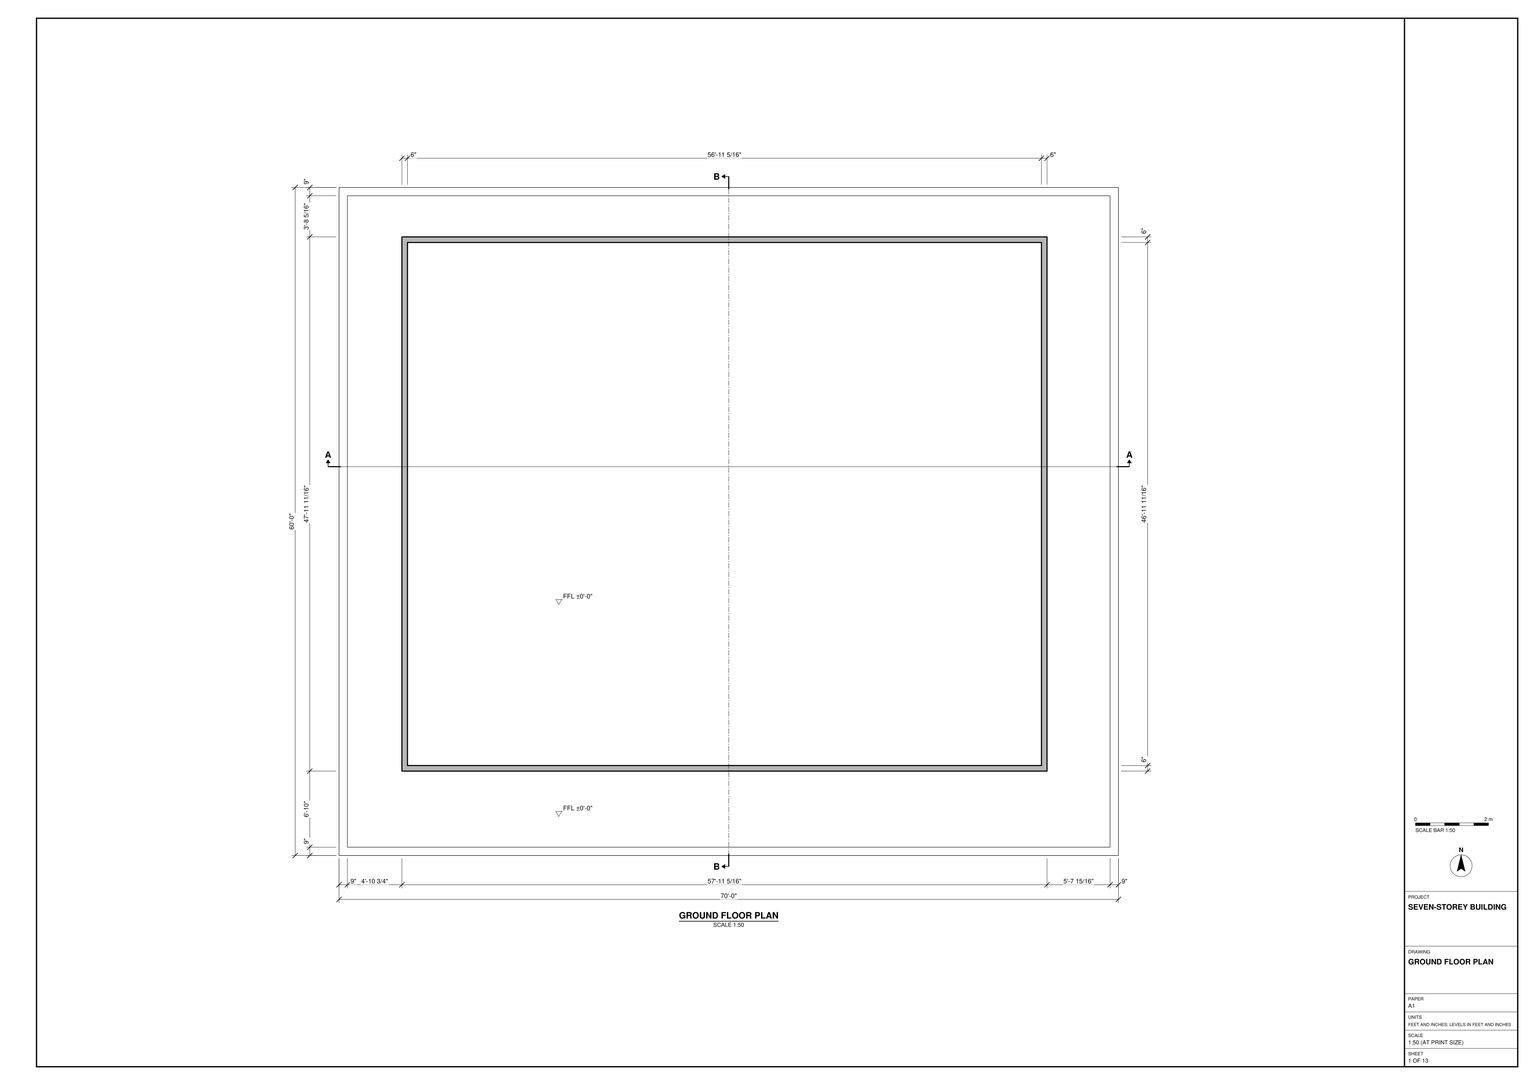
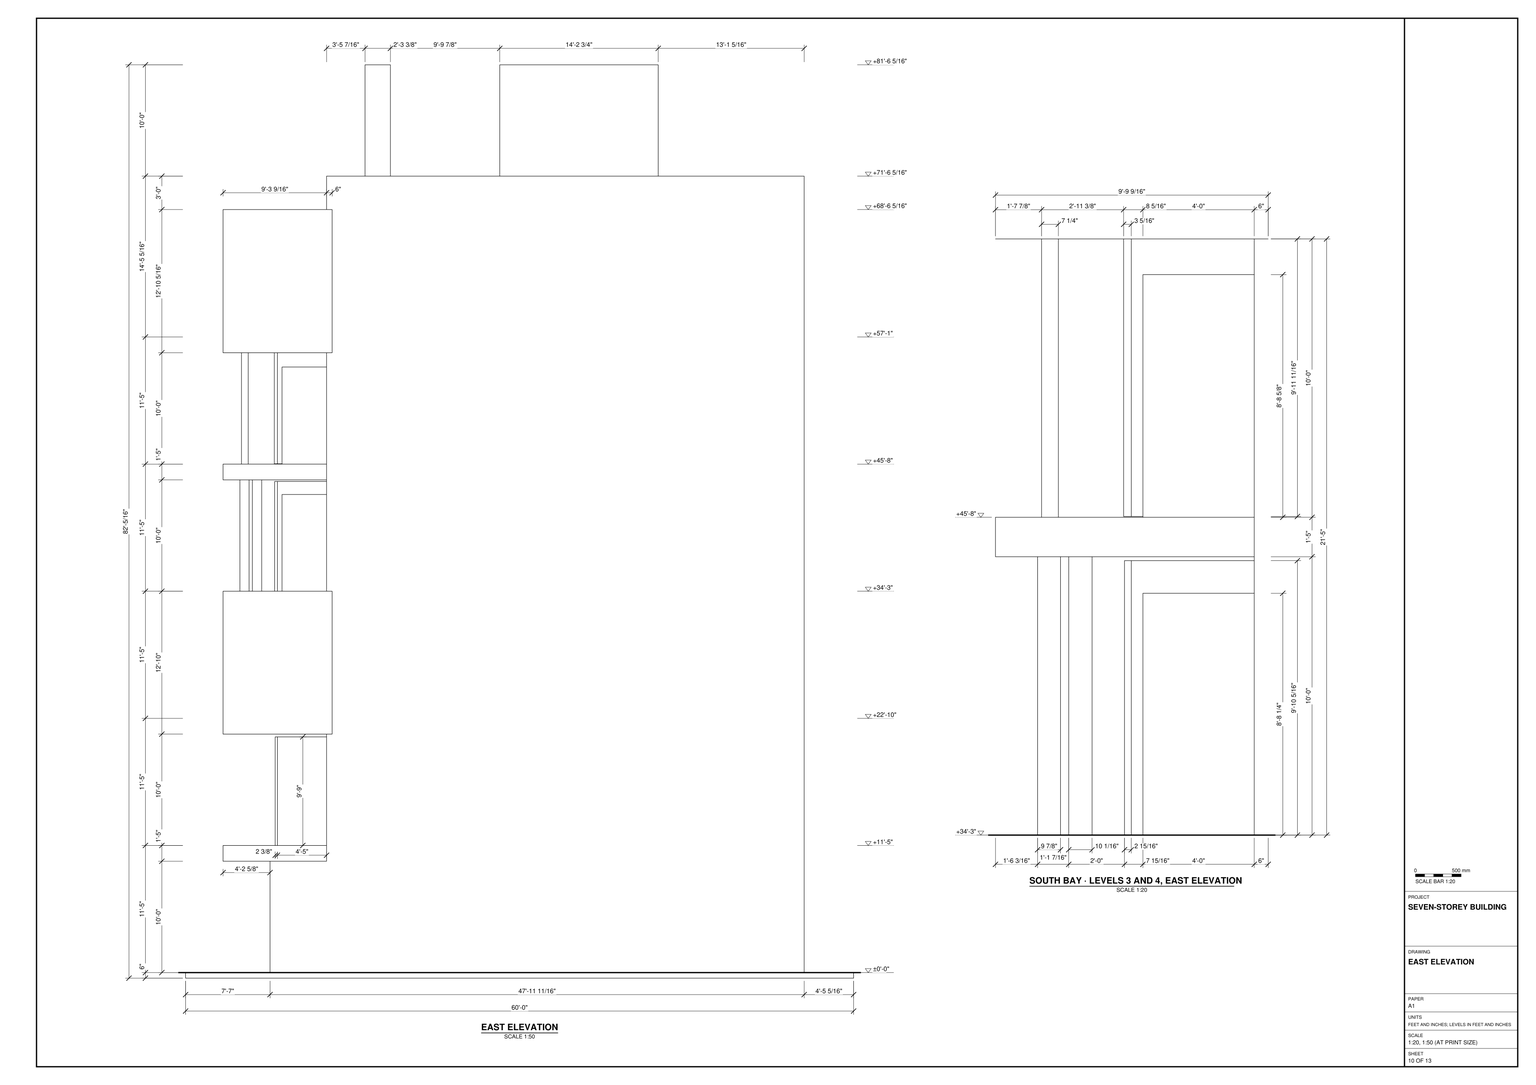
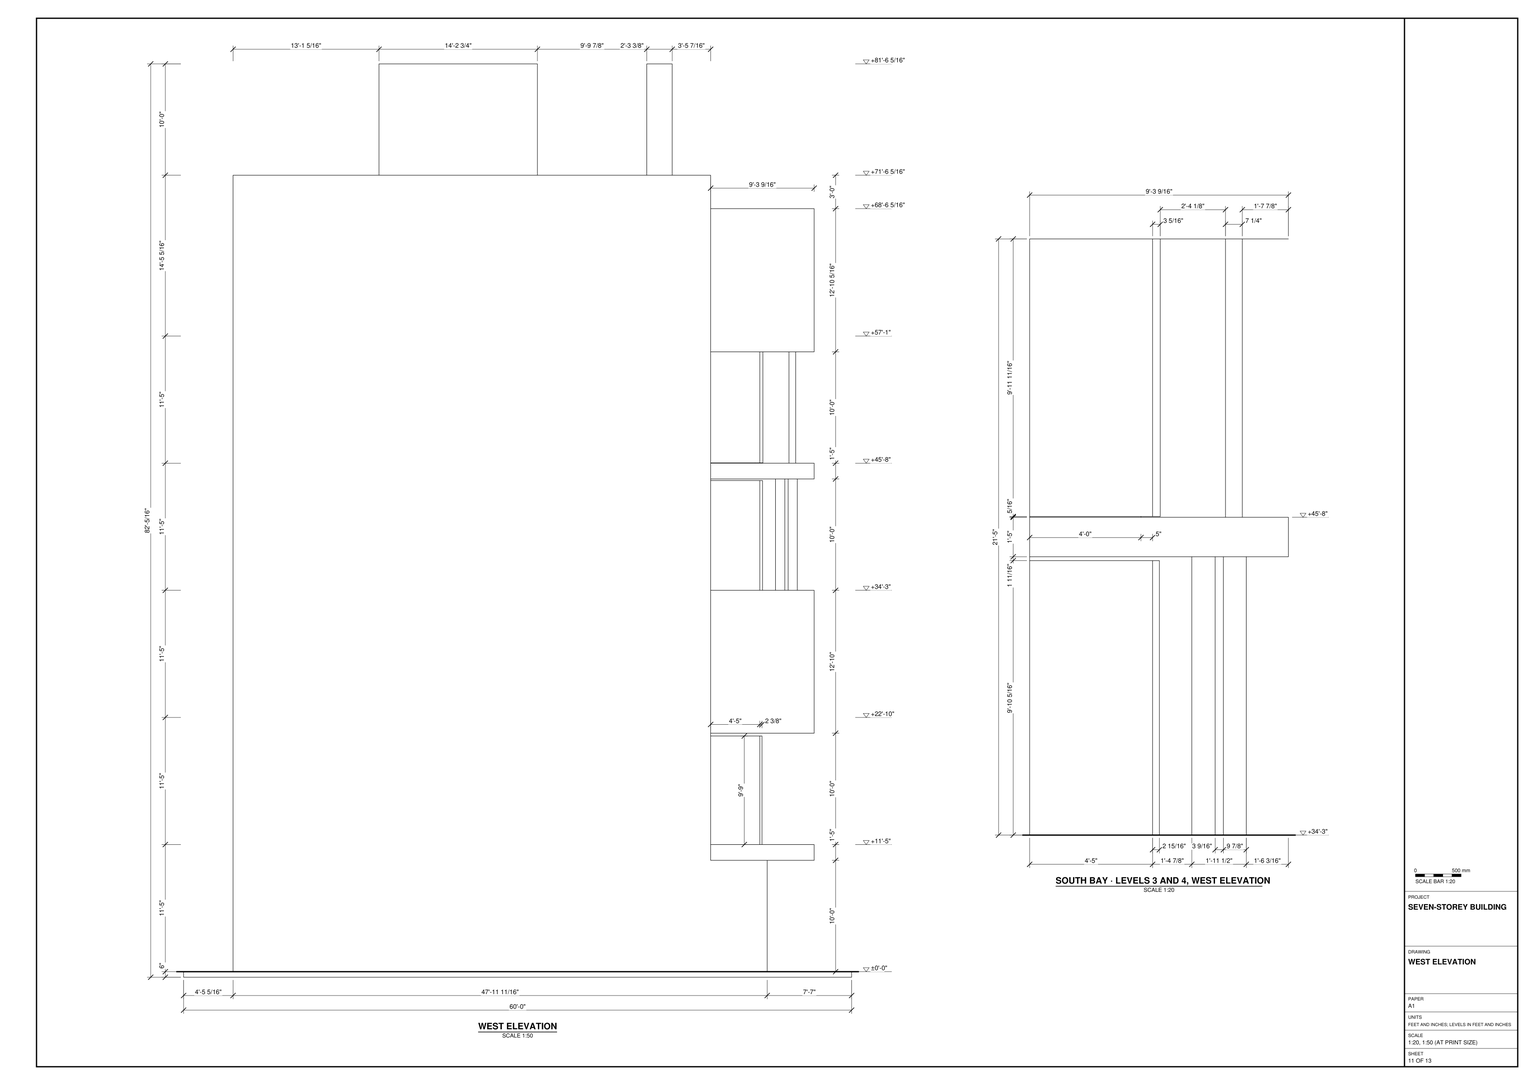
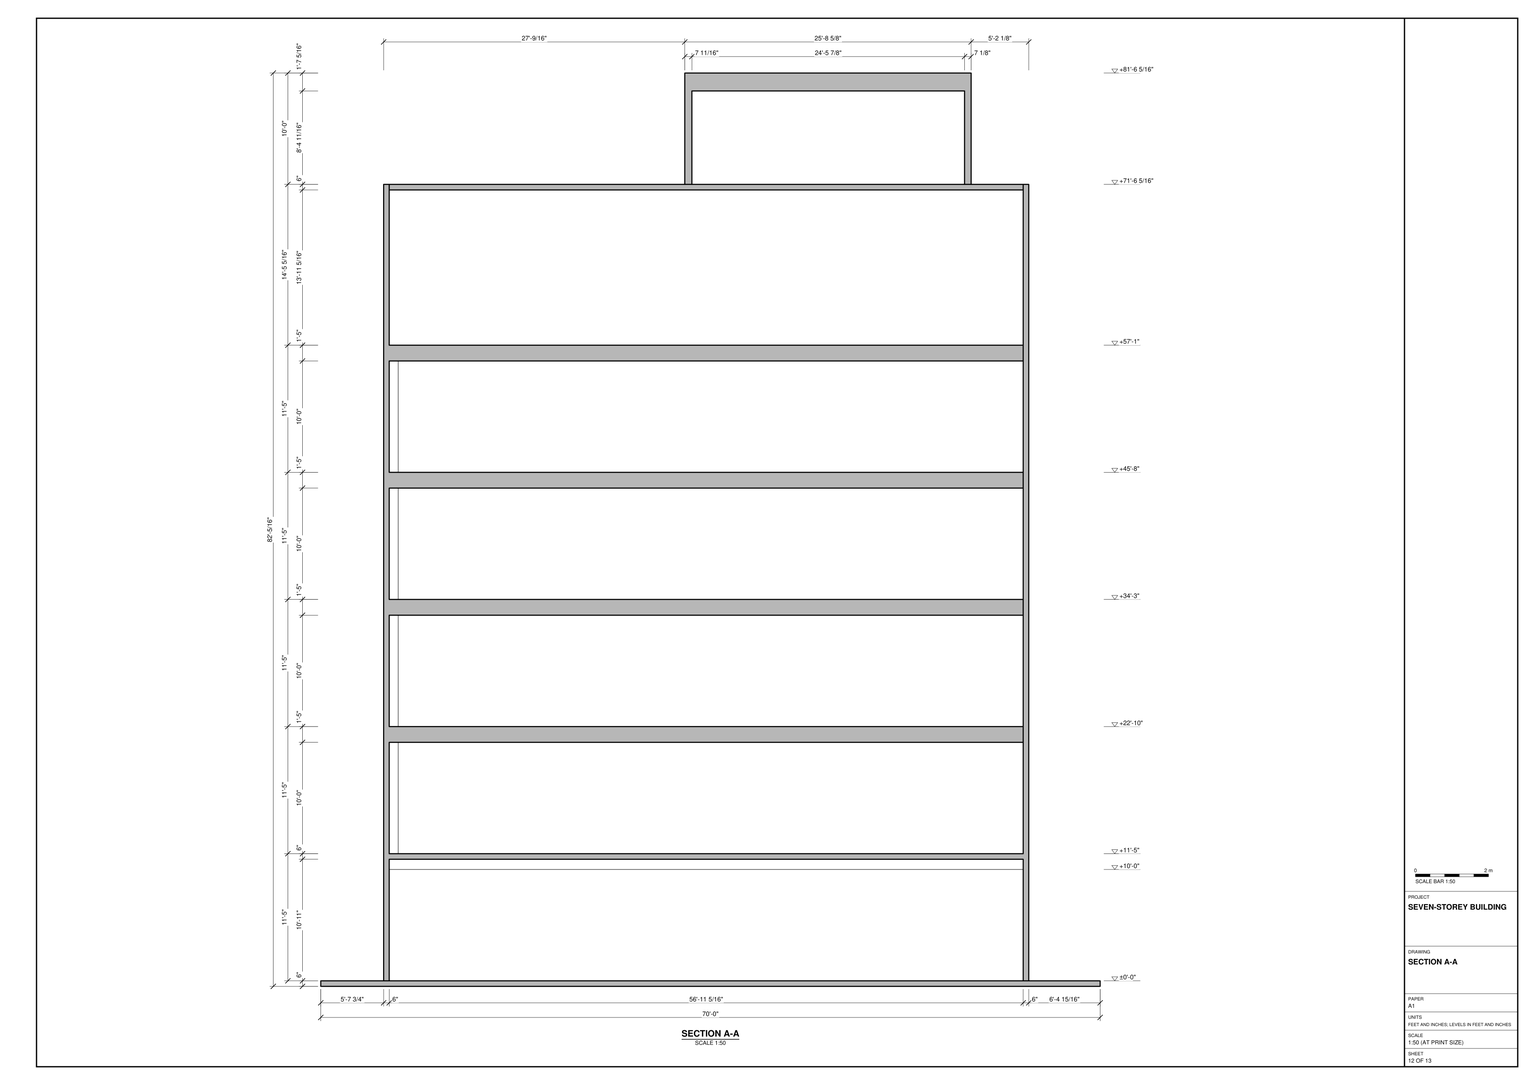
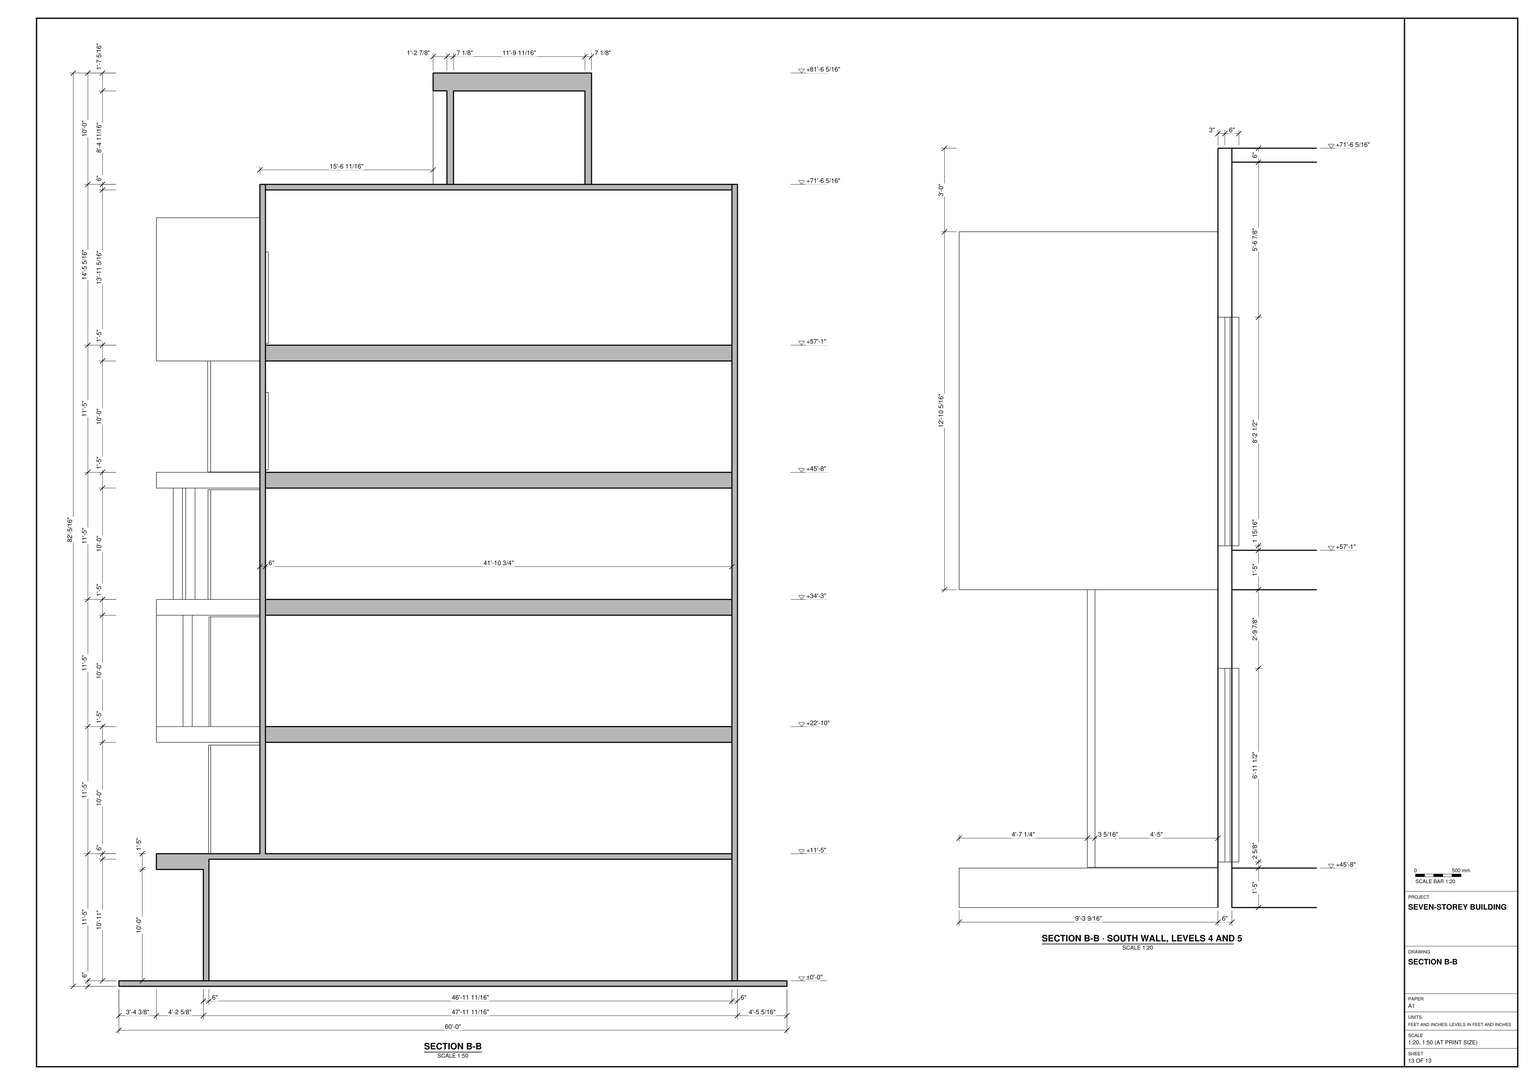
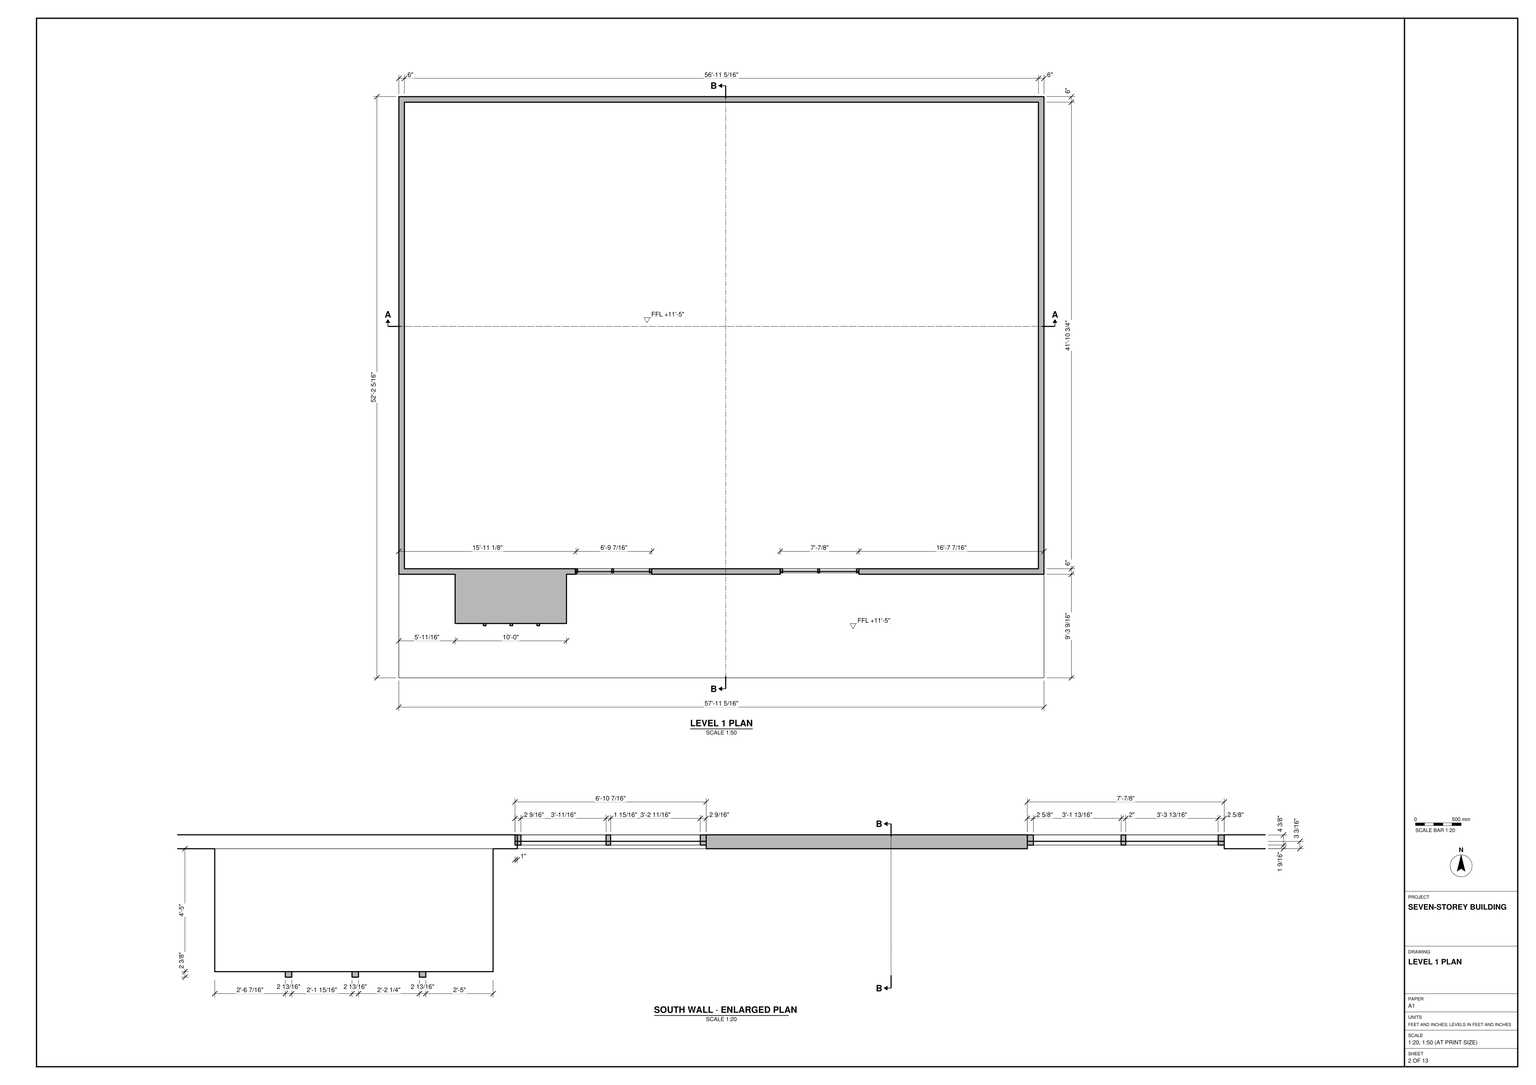
Build the seven-storey building in SketchUp from task_files/diagram_01.pdf. Work in feet and inches. The overall model is 70'-0" east to west, 60'-0" north to south and 82'-5/16" high. Set the levels, relative to the ground floor, at ±0'-0", +11'-5", +22'-10", +34'-3", +45'-8", +57'-1" and +71'-6 5/16".

Start with the thin rectangular base. Set out the ground-floor walls from the dimensioned offsets on the plan rather than centring the footprint on the base. Keep the open interior shown on that plan and give the walls their drawn thicknesses. Follow the plans and sections for floor slabs, openings, stairs and roof geometry. Model built-in joinery and main furniture only where shown.

Use the east and west elevations to shape the south side: the upper wall line steps back from the ground floor, while the bays project beyond it. Distinguish the solid-sided portions from the open portions with slender uprights and projecting slab edges. Use the enlarged bay elevations for the placement of those uprights. Include the raised forms above the main roof in their drawn positions.

Keep shell elements such as walls, slabs and roof separate as groups or components. Group each furniture or joinery piece separately and use components for repeated parts. Any decor or loose items shown may be represented by suitable library components. Save one SketchUp model as output_files/seven_storey_building_with_projecting_south_bays.skp.

# SketchUp Ruby script. Lengths in inches.
U = 1.inch
M = Sketchup.active_model
def pt(a) = Geom::Point3d.new(a.map { |v| v * U })
def face(e, loops, mat)
  f = e.add_face(loops[0].map { |a| pt(a) })
  loops[1..].each { |l| e.add_face(l.map { |a| pt(a) }).erase! }
  f.material = f.back_material = mat if mat
  f
end
# faces: each face lists its corners as indices into pts; further lists are holes
def faces(e, pts, list, mat = nil) = list.each { |f| face(e, (f[0].is_a?(Array) ? f : [f]).map { |l| l.map { |i| pts[i] } }, mat) }
# xy, xz, yz: faces in a plane at the given z, y or x. An outline is a flat list of corners, or four numbers for a rectangle; further outlines are holes
def ring(l) = l.size == 4 ? [[l[0], l[1]], [l[2], l[1]], [l[2], l[3]], [l[0], l[3]]] : l.each_slice(2).to_a
def flat(e, list, mat, &to3) = list.each { |f| face(e, (f[0].is_a?(Array) ? f : [f]).map { |l| ring(l).map { |u, v| to3.(u, v) } }, mat) }
def xy(e, z, list, mat = nil) = flat(e, list, mat) { |x, y| [x, y, z] }
def xz(e, y, list, mat = nil) = flat(e, list, mat) { |x, z| [x, y, z] }
def yz(e, x, list, mat = nil) = flat(e, list, mat) { |y, z| [x, y, z] }
def lines(e, pts, list) = list.each { |a, b| e.add_line(pt(pts[a]), pt(pts[b])) }
# prism: a flat outline (further loops are holes) pulled along v
def prism(e, loops, v, mat = nil)
  f = face(e, loops, mat); d = Geom::Vector3d.new(v.map { |x| x * U })
  f.pushpull(f.normal.samedirection?(d) ? d.length : -d.length)
end
def box(e, o, s, mat = nil) = prism(e, [[o, [o[0] + s[0], o[1], o[2]], [o[0] + s[0], o[1] + s[1], o[2]], [o[0], o[1] + s[1], o[2]]]], [0, 0, s[2]], mat)
def at(x, y, z, deg = 0) = Geom::Transformation.translation(pt([x, y, z])) * Geom::Transformation.rotation(ORIGIN, Z_AXIS, deg.degrees)
def axes(o, x, y, z) = Geom::Transformation.new([*x, 0, *y, 0, *z, 0, *pt(o).to_a, 1])
def part(name) = M.definitions.add(name)
# library, detail: a bought-in or finely detailed component or shape, given as its bounding box
def library(name, o, s) = part(name).tap { |d| box(d.entities, o, s) }
def detail(e, o, s) = box(e.add_group.entities, o, s)
def put(e, d, t, mat = nil) = e.add_instance(d, t).tap { |i| i.material = mat if mat }
def group(e, t, mat = nil) = e.add_group.tap { |g| g.transformation = t; g.material = mat if mat }.entities
root = M.entities
M.materials.add("[0012_Bisque]").color = [255, 228, 196]
M.materials.add("[0131_Silver]").color = [192, 192, 192]
M.materials.add("[Color B08]").color = [102, 25, 0]
M.materials.add("[Color D01]").color = [255, 242, 204]
M.materials.add("[Color E01]").color = [255, 255, 204]
M.materials.add("[Color M03]").color = [170, 170, 170]
M.materials.add("[Color M04]").color = [142, 142, 142]
M.materials.add("[Mirror 02]").color = [229, 229, 229]
M.materials.add("[Stone Masonry Multi]").color = [182, 175, 164]
M.materials.add("[Translucent Glass Gray]").color = [128, 128, 128]
M.materials["[Translucent Glass Gray]"].alpha = 0.5
M.materials.add("[Wood Board Cork]").color = [233, 201, 166]
c1 = part("Group\#1")
xy(c1.entities,0,[[0,0,65.9375,1.625],[0,1.625,65.9375,4.375]],"[Color B08]")
xy(c1.entities,2.04,[[2.04,0,31.4,1.625],[32.97,0,63.9,1.625],[2.04,1.625,31.4,4.375],[32.97,1.625,63.9,4.375]],"[Color B08]")
xy(c1.entities,48.03,[[2.04,0,31.4,1.625],[32.97,0,63.9,1.625],[2.04,1.625,31.4,4.375],[32.97,1.625,63.9,4.375]],"[Color B08]")
xy(c1.entities,50.0625,[[0,0,65.9375,1.625],[0,1.625,65.9375,4.375]],"[Color B08]")
xz(c1.entities,0,[[[0,0,65.9375,50.0625],[32.97,2.04,63.9,48.03],[2.04,2.04,31.4,48.03]]],"[Color B08]")
xz(c1.entities,1.625,[[[0,0,65.9375,50.0625],[32.97,2.04,63.9,48.03],[2.04,2.04,31.4,48.03]]],"[Color B08]")
xz(c1.entities,1.625,[[2.04,2.04,31.4,48.03],[32.97,2.04,63.9,48.03]],"[Translucent Glass Gray]")
xz(c1.entities,4.375,[[[0,0,65.9375,50.0625],[32.97,2.04,63.9,48.03],[2.04,2.04,31.4,48.03]]],"[Color B08]")
yz(c1.entities,0,[[0,0,1.625,50.0625],[1.625,0,4.375,50.0625]],"[Color B08]")
yz(c1.entities,2.04,[[0,2.04,1.625,48.03],[1.625,2.04,4.375,48.03]],"[Color B08]")
yz(c1.entities,31.4,[[0,2.04,1.625,48.03],[1.625,2.04,4.375,48.03]],"[Color B08]")
yz(c1.entities,32.97,[[0,2.04,1.625,48.03],[1.625,2.04,4.375,48.03]],"[Color B08]")
yz(c1.entities,63.9,[[0,2.04,1.625,48.03],[1.625,2.04,4.375,48.03]],"[Color B08]")
yz(c1.entities,65.9375,[[0,0,1.625,50.0625],[1.625,0,4.375,50.0625]],"[Color B08]")
xy(root,0,[[0,0,840,720]])
xy(root,6,[[[0,0,840,720],[9,9,831,711]],[[9,9,831,711],[67.75,91,763.0625,666.6875]],[[67.75,91,763.0625,666.6875],[73.75,97,757.0625,660.6875]],[73.75,97,757.0625,660.6875]])
xy(root,126,[[67.75,40.375,763.0625,91]],"[Color M04]")
xy(root,137,[[73.75,97,757.0625,660.6875]])
xy(root,143,[[563.63,151.9375,757.0625,157.9375],[73.75,157.9375,757.0625,660.6875]])
xy(root,143,[[158.84,96.5625,161.63,98.9375],[187.59,96.5625,190.38,98.9375],[216.61,96.5625,219.4,98.9375]],"[Color B08]")
xy(root,143,[[67.75,40.375,763.0625,40.375,763.0625,151.9375,563.63,151.9375,563.63,157.9375,478.75,157.9375,478.75,151.9375,248.42,151.9375,248.42,98.9375,219.4,98.9375,219.4,96.5625,216.61,96.5625,216.61,98.9375,190.38,98.9375,190.38,96.5625,187.59,96.5625,187.59,98.9375,161.63,98.9375,161.63,96.5625,158.84,96.5625,158.84,98.9375,128.42,98.9375,128.42,151.9375,67.75,151.9375]],"[Color M04]")
xy(root,145.06,[[258.86,151.9375,340.3,157.9375]])
xy(root,230.99,[[258.86,151.9375,340.3,157.9375]])
xy(root,245.625,[[478.75,151.9375,563.63,157.9375]])
xy(root,260,[[128.42,98.9375,248.42,151.9375]])
xy(root,260,[[158.84,96.5625,161.63,98.9375],[187.59,96.5625,190.38,98.9375],[216.61,96.5625,219.4,98.9375]],"[Color B08]")
xy(root,263,[[757.0625,151.9375,763.0625,157.9375],[73.75,157.9375,757.0625,660.6875]])
xy(root,263,[[67.75,40.375,368.67,151.9375],[458.5,40.375,763.0625,151.9375]],"[Color M04]")
xy(root,280,[[166.18,69.12,205.99,79],[615.32,69.47,664.01,89.59],[567.24,71.3,578.86,84.99],[583.61,71.3,595.24,84.99],[599.99,71.3,611.61,84.99],
  [128.42,98.9375,248.42,151.9375],[73.75,157.9375,757.0625,660.6875]])
xy(root,280,[[157.2,97.125,159.26,98.9375],[186.95,97.125,189.01,98.9375],[216.65,97.125,218.72,98.9375]],"[Color B08]")
xy(root,280,[[[83.875,40.375,368.67,40.375,368.67,151.9375,248.42,151.9375,248.42,98.9375,218.72,98.9375,218.72,97.125,216.65,97.125,216.65,98.9375,189.01,98.9375,189.01,97.125,186.95,97.125,186.95,98.9375,159.26,98.9375,159.26,97.125,157.2,97.125,157.2,98.9375,128.42,98.9375,128.42,151.9375,83.875,151.9375],[166.18,69.12,205.99,79]],[[458.5,40.375,746.875,40.375,746.875,151.9375,563.63,151.9375,563.63,157.9375,478.75,157.9375,478.75,151.9375,458.5,151.9375],[615.32,69.47,664.01,89.59],[599.99,71.3,611.61,84.99],[583.61,71.3,595.24,84.99],[567.24,71.3,578.86,84.99]]],"[Color E01]")
xy(root,284.24,[[258.86,151.9375,340.3,157.9375]])
xy(root,371.93,[[258.86,151.9375,340.3,157.9375]])
xy(root,382.125,[[478.75,151.9375,563.63,157.9375]])
xy(root,398.25,[[128.42,98.9375,248.42,151.9375]])
xy(root,398.25,[[157.2,97.125,159.26,98.9375],[186.95,97.125,189.01,98.9375],[216.65,97.125,218.72,98.9375]],"[Color B08]")
xy(root,400,[[73.75,157.9375,757.0625,660.6875]])
xy(root,400,[[[83.875,40.375,368.67,151.9375],[166.18,69.12,205.99,79]],[[458.5,40.375,746.875,151.9375],[615.32,69.47,664.01,89.59],[599.99,71.3,611.61,84.99],[583.61,71.3,595.24,84.99],[567.24,71.3,578.86,84.99]]],"[Color E01]")
xy(root,417,[[166.18,58.54,205.99,68.42],[132.64,71.97,240.64,82.03],[128.42,98.9375,248.42,151.9375],[757.0625,151.9375,763.0625,157.9375],[73.75,157.9375,757.0625,660.6875]])
xy(root,417,[[151.95,96,154.09,98.9375],[178.52,96,180.65,98.9375],[209.39,96,211.53,98.9375]],"[Color B08]")
xy(root,417,[[[67.75,40.375,368.67,40.375,368.67,151.9375,248.42,151.9375,248.42,98.9375,211.53,98.9375,211.53,96,209.39,96,209.39,98.9375,180.65,98.9375,180.65,96,178.52,96,178.52,98.9375,154.09,98.9375,154.09,96,151.95,96,151.95,98.9375,128.42,98.9375,128.42,151.9375,67.75,151.9375],[132.64,71.97,240.64,82.03],[166.18,58.54,205.99,68.42]],[458.5,40.375,763.0625,40.375,763.0625,151.9375,733.02,151.9375,733.02,103.9375,608.71,103.9375,608.71,151.9375,563.63,151.9375,563.63,157.9375,478.75,157.9375,478.75,151.9375,458.5,151.9375]],"[Color M04]")
xy(root,421.06,[[258.86,151.9375,340.3,157.9375]])
xy(root,506.37,[[258.86,151.9375,340.3,157.9375]])
xy(root,521.25,[[608.71,103.9375,733.02,151.9375]])
xy(root,521.6875,[[478.75,151.9375,563.63,157.9375]])
xy(root,535.3125,[[128.42,98.9375,248.42,151.9375]])
xy(root,535.3125,[[151.95,96,154.09,98.9375],[178.52,96,180.65,98.9375],[209.39,96,211.53,98.9375]],"[Color B08]")
xy(root,537,[[73.75,157.9375,757.0625,660.6875]])
xy(root,537,[[[67.75,40.375,368.67,151.9375],[132.64,71.97,240.64,82.03],[166.18,58.54,205.99,68.42]],[458.5,40.375,763.0625,151.9375]],"[Color M04]")
xy(root,554,[[495.52,60.25,500.52,67.5],[503.08,60.25,508.08,67.5],[510.4,60.25,515.4,67.5],[668.58,60.25,673.58,67.5],[676.08,60.25,681.08,67.5],
  [683.77,60.25,688.77,67.5],[692.21,60.25,697.21,67.5],[700.65,60.25,705.65,67.5],[73.75,157.9375,757.0625,660.6875]])
xy(root,554,[[67.75,40.375,368.67,151.9375],[[458.5,40.375,763.0625,40.375,763.0625,151.9375,733.02,151.9375,733.02,103.9375,608.71,103.9375,608.71,151.9375,563.63,151.9375,563.63,157.9375,478.75,157.9375,478.75,151.9375,458.5,151.9375],[495.52,60.25,500.52,67.5],[503.08,60.25,508.08,67.5],[510.4,60.25,515.4,67.5],[668.58,60.25,673.58,67.5],[676.08,60.25,681.08,67.5],[683.77,60.25,688.77,67.5],[692.21,60.25,697.21,67.5],[700.65,60.25,705.65,67.5]]],"[Color M04]")
xy(root,554.34,[[128.42,98.9375,248.42,151.9375]])
xy(root,554.34,[[158.47,95.625,161.56,98.9375],[187.16,95.625,190.25,98.9375],[216.53,95.625,219.62,98.9375]],"[Color B08]")
xy(root,556.62,[[258.86,151.9375,340.3,157.9375]])
xy(root,640.12,[[258.86,151.9375,340.3,157.9375]])
xy(root,657.125,[[478.75,151.9375,563.63,157.9375]])
xy(root,658.62,[[608.71,103.9375,733.02,151.9375]])
xy(root,674,[[128.42,98.9375,248.42,151.9375],[757.0625,151.9375,763.0625,157.9375],[73.75,157.9375,757.0625,660.6875]])
xy(root,674,[[158.47,95.625,161.56,98.9375],[187.16,95.625,190.25,98.9375],[216.53,95.625,219.62,98.9375]],"[Color B08]")
xy(root,674,[[67.75,40.375,67.75,151.9375,128.42,151.9375,128.42,98.9375,158.47,98.9375,158.47,95.625,161.56,95.625,161.56,98.9375,187.16,98.9375,187.16,95.625,190.25,95.625,190.25,98.9375,216.53,98.9375,216.53,95.625,219.62,95.625,219.62,98.9375,248.42,98.9375,248.42,151.9375,368.67,151.9375,368.67,40.375],[[458.5,40.375,763.0625,151.9375],[700.65,60.25,705.65,67.5],[668.58,60.25,673.58,67.5],[676.08,60.25,681.08,67.5],[683.77,60.25,688.77,67.5],[692.21,60.25,697.21,67.5],[503.08,60.25,508.08,67.5],[495.52,60.25,500.52,67.5],[510.4,60.25,515.4,67.5]]],"[Color M04]")
xy(root,691,[[605.05,58.7,649.17,75.51],[174.62,61.6,211.18,73.72],[567.68,65.39,574.43,72.14],[577.49,65.39,584.24,72.14],[587.3,65.39,594.05,72.14],
  [597.11,65.39,603.86,72.14],[126.47,98.9375,246.47,151.9375],[73.75,157.9375,757.0625,660.6875]])
xy(root,691,[[157.25,96.6875,159.45,98.9375],[189.56,96.6875,191.76,98.9375],[217.06,96.6875,219.26,98.9375]],"[Color B08]")
xy(root,691,[[[83.875,40.375,353.79,40.375,353.79,151.9375,246.47,151.9375,246.47,98.9375,219.26,98.9375,219.26,96.6875,217.06,96.6875,217.06,98.9375,191.76,98.9375,191.76,96.6875,189.56,96.6875,189.56,98.9375,159.45,98.9375,159.45,96.6875,157.25,96.6875,157.25,98.9375,126.47,98.9375,126.47,151.9375,83.875,151.9375],[174.62,61.6,211.18,73.72]],[[474.79,40.375,746.875,40.375,746.875,151.9375,733.02,151.9375,733.02,103.9375,608.71,103.9375,608.71,151.9375,563.63,151.9375,563.63,157.9375,478.75,157.9375,478.75,151.9375,474.79,151.9375],[605.05,58.7,649.17,75.51],[597.11,65.39,603.86,72.14],[587.3,65.39,594.05,72.14],[577.49,65.39,584.24,72.14],[567.68,65.39,574.43,72.14]]],"[Color E01]")
xy(root,692.93,[[258.86,151.9375,340.3,157.9375]])
xy(root,791.43,[[258.86,151.9375,340.3,157.9375]])
xy(root,795,[[478.75,151.9375,563.63,157.9375]])
xy(root,796.37,[[608.71,103.9375,733.02,151.9375]])
xy(root,811,[[126.47,98.9375,246.47,151.9375]])
xy(root,811,[[157.25,96.6875,159.45,98.9375],[189.56,96.6875,191.76,98.9375],[217.06,96.6875,219.26,98.9375]],"[Color B08]")
xy(root,811,[[[83.875,40.375,83.875,151.9375,126.47,151.9375,126.47,98.9375,157.25,98.9375,157.25,96.6875,159.45,96.6875,159.45,98.9375,189.56,98.9375,189.56,96.6875,191.76,96.6875,191.76,98.9375,217.06,98.9375,217.06,96.6875,219.26,96.6875,219.26,98.9375,246.47,98.9375,246.47,151.9375,353.79,151.9375,353.79,40.375],[174.62,61.6,211.18,73.72]],[[474.79,40.375,746.875,151.9375],[605.05,58.7,649.17,75.51],[567.68,65.39,574.43,72.14],[577.49,65.39,584.24,72.14],[587.3,65.39,594.05,72.14],[597.11,65.39,603.86,72.14]]],"[Color E01]")
xy(root,828.3125,[[757.0625,151.9375,763.0625,157.9375]])
xy(root,828.3125,[[67.75,40.375,368.67,151.9375],[458.5,40.375,763.0625,151.9375]],"[Color M04]")
xy(root,858.3125,[[73.75,157.9375,757.0625,660.6875]])
xy(root,864.3125,[[67.75,151.9375,757.0625,151.9375,757.0625,157.9375,73.75,157.9375,73.75,660.6875,757.0625,660.6875,757.0625,151.9375,763.0625,151.9375,763.0625,666.6875,67.75,666.6875],[[73.75,157.9375,757.0625,660.6875],[392.33,338.63,392.33,509.38,700.96,509.38,700.96,338.63,693.86,338.63,693.86,353.51,399.99,353.51,399.99,338.63],[429.77,193.39,659.52,220.76]],[429.77,193.39,659.52,220.76],[[392.33,338.63,392.33,509.38,700.96,509.38,700.96,338.63,693.86,338.63,693.86,353.51,399.99,353.51,399.99,338.63],[399.99,360.6,693.86,502.29]],[399.99,360.6,693.86,502.29]])
xy(root,868.17,[[433.625,193.39,655.67,197.64]],"[Stone Masonry Multi]")
xy(root,965,[[399.99,360.6,693.86,502.29]])
xy(root,965.12,[[399.99,338.63,693.86,353.51]])
xy(root,980.46,[[433.625,193.39,655.67,197.64]],"[Stone Masonry Multi]")
xy(root,984.3125,[[392.33,338.63,700.96,509.38]],"[Color D01]")
xy(root,984.3125,[[429.77,193.39,659.52,220.76]],"[Stone Masonry Multi]")
xz(root,0,[[0,0,840,6]])
xz(root,40.375,[[67.75,126,763.0625,143],[67.75,263,368.67,263,368.67,280,83.875,280,83.875,400,368.67,400,368.67,417,67.75,417],[458.5,263,763.0625,263,763.0625,417,458.5,417,458.5,400,746.875,400,746.875,280,458.5,280],[67.75,537,368.67,554],[458.5,537,763.0625,554],
  [[67.75,674,368.67,828.3125],[83.875,691,353.79,811]],[[458.5,674,763.0625,828.3125],[474.79,691,746.875,811]]],"[Color M04]")
xz(root,58.54,[[166.18,417,205.99,537]],"[Stone Masonry Multi]")
xz(root,58.7,[[605.05,691,649.17,811]],"[Stone Masonry Multi]")
xz(root,60.25,[[495.52,554,500.52,674],[503.08,554,508.08,674],[510.4,554,515.4,674],[668.58,554,673.58,674],[676.08,554,681.08,674],
  [683.77,554,688.77,674],[692.21,554,697.21,674],[700.65,554,705.65,674]],"[Wood Board Cork]")
xz(root,61.6,[[174.62,691,181.51,811],[181.51,691,188.45,811],[188.45,691,194.83,811],[194.83,691,201.89,811],[201.89,691,211.18,811]],"[Wood Board Cork]")
xz(root,65.39,[[567.68,691,574.43,811],[577.49,691,584.24,811],[587.3,691,594.05,811],[597.11,691,603.86,811]],"[Wood Board Cork]")
xz(root,67.5,[[495.52,554,500.52,674],[503.08,554,508.08,674],[510.4,554,515.4,674],[668.58,554,673.58,674],[676.08,554,681.08,674],
  [683.77,554,688.77,674],[692.21,554,697.21,674],[700.65,554,705.65,674]],"[Wood Board Cork]")
xz(root,68.42,[[166.18,417,205.99,537]])
xz(root,69.12,[[166.18,280,205.99,400]],"[Stone Masonry Multi]")
xz(root,69.47,[[615.32,280,664.01,400]],"[Stone Masonry Multi]")
xz(root,71.3,[[567.24,280,578.86,400],[583.61,280,595.24,400],[599.99,280,611.61,400]],"[Wood Board Cork]")
xz(root,71.97,[[179.93,417,186.74,537],[186.74,417,193.55,537],[193.55,417,200.36,537]])
xz(root,71.97,[[132.64,417,139.05,537],[139.05,417,145.86,537],[145.86,417,152.68,537],[152.68,417,159.49,537],[159.49,417,166.3,537],
  [166.3,417,173.11,537],[173.11,417,179.93,537],[200.36,417,207.18,537],[207.18,417,213.99,537],[213.99,417,220.8,537],
  [220.8,417,227.61,537],[227.61,417,234.43,537],[234.43,417,240.64,537]],"[Wood Board Cork]")
xz(root,72.14,[[567.68,691,574.43,811],[577.49,691,584.24,811],[587.3,691,594.05,811],[597.11,691,603.86,811]],"[Wood Board Cork]")
xz(root,73.72,[[174.62,691,211.18,811]],"[Wood Board Cork]")
xz(root,75.51,[[605.05,691,649.17,811]],"[Stone Masonry Multi]")
xz(root,79,[[166.18,280,205.99,400]],"[Stone Masonry Multi]")
xz(root,82.03,[[132.64,417,240.64,537]],"[Wood Board Cork]")
xz(root,84.99,[[567.24,280,578.86,400],[583.61,280,595.24,400],[599.99,280,611.61,400]],"[Wood Board Cork]")
xz(root,89.59,[[615.32,280,664.01,400]],"[Stone Masonry Multi]")
xz(root,91,[[67.75,6,763.0625,126]],"[Color M03]")
xz(root,95.625,[[158.47,554.34,161.56,674],[187.16,554.34,190.25,674],[216.53,554.34,219.62,674]],"[Color B08]")
xz(root,96,[[151.95,417,154.09,535.3125],[178.52,417,180.65,535.3125],[209.39,417,211.53,535.3125]],"[Color B08]")
xz(root,96.5625,[[158.84,143,161.63,260],[187.59,143,190.38,260],[216.61,143,219.4,260]],"[Color B08]")
xz(root,96.6875,[[157.25,691,159.45,811],[189.56,691,191.76,811],[217.06,691,219.26,811]],"[Color B08]")
xz(root,97,[[73.75,6,757.0625,126],[73.75,126,757.0625,137]])
xz(root,97.125,[[157.2,280,159.26,398.25],[186.95,280,189.01,398.25],[216.65,280,218.72,398.25]],"[Color B08]")
xz(root,98.9375,[[158.84,143,161.63,260],[187.59,143,190.38,260],[216.61,143,219.4,260],[157.2,280,159.26,398.25],[186.95,280,189.01,398.25],
  [216.65,280,218.72,398.25],[151.95,417,154.09,535.3125],[178.52,417,180.65,535.3125],[209.39,417,211.53,535.3125],[158.47,554.34,161.56,674],
  [187.16,554.34,190.25,674],[216.53,554.34,219.62,674],[157.25,691,159.45,811],[189.56,691,191.76,811],[217.06,691,219.26,811]],"[Color B08]")
xz(root,98.9375,[[128.42,143,158.84,260],[161.63,143,187.59,260],[190.38,143,216.61,260],[219.4,143,248.42,260],[128.42,280,157.2,398.25],
  [159.26,280,186.95,398.25],[189.01,280,216.65,398.25],[218.72,280,248.42,398.25],[128.42,417,151.95,535.3125],[154.09,417,178.52,535.3125],
  [180.65,417,209.39,535.3125],[211.53,417,248.42,535.3125],[128.42,554.34,158.47,674],[161.56,554.34,187.16,674],[190.25,554.34,216.53,674],
  [219.62,554.34,248.42,674],[126.47,691,157.25,811],[159.45,691,189.56,811],[191.76,691,217.06,811],[219.26,691,246.47,811]],"[Mirror 02]")
xz(root,103.9375,[[608.71,691,630.91,796.37]])
xz(root,103.9375,[[635.22,417,638.14,521.25],[663.78,417,666.7,521.25],[696.41,417,699.33,521.25],[634.36,554,636.13,658.62],[663.17,554,664.94,658.62],
  [630.91,691,633.55,691,633.55,745.62,680.03,745.62,680.03,691,682.68,691,682.68,745.62,733.02,745.62,733.02,748.15,682.68,748.15,682.68,796.37,680.03,796.37,680.03,748.15,633.55,748.15,633.55,796.37,630.91,796.37]],"[Color B08]")
xz(root,103.9375,[[608.71,417,635.22,521.25],[638.14,417,663.78,521.25],[666.7,417,696.41,521.25],[699.33,417,733.02,521.25],[608.71,554,634.36,658.62],
  [636.13,554,663.17,658.62],[664.94,554,733.02,658.62],[633.55,691,680.03,745.62],[682.68,691,733.02,745.62],[633.55,748.15,680.03,796.37],
  [682.68,748.15,733.02,796.37]],"[Mirror 02]")
xz(root,151.9375,[[128.42,260,248.42,260.34],[67.75,263,73.75,280],[73.75,263,73.75,280,128.42,280,128.42,278.59,248.42,278.59,248.42,280,368.67,280,368.67,263],[458.5,263,458.5,280,478.75,280,478.75,279.5,563.63,279.5,563.63,280,757.0625,280,757.0625,263],[128.42,278.59,248.42,280],
  [67.75,280,83.875,400],[746.875,280,757.0625,400],[128.42,398.25,248.42,398.59],[67.75,400,73.75,417],[73.75,400,73.75,417,128.42,417,128.42,415.66,248.42,415.66,248.42,417,368.67,417,368.67,400],
  [128.42,415.66,248.42,417],[128.42,535.3125,248.42,535.66],[67.75,537,368.67,554],[67.75,674,67.75,828.3125,73.75,828.3125,73.75,811,83.875,811,83.875,691,73.75,691,73.75,674],[73.75,674,73.75,691,368.67,691,368.67,674,248.42,674,248.42,674.34,128.42,674.34,128.42,674],
  [128.42,674,248.42,674.34],[353.79,691,368.67,811],[458.5,691,474.79,811],[746.875,691,757.0625,811],[73.75,811,368.67,828.3125],
  [458.5,811,757.0625,828.3125]])
xz(root,151.9375,[[[67.75,143,128.42,143,128.42,260.34,248.42,260.34,248.42,143,368.67,143,368.67,263,67.75,263],[258.86,145.06,340.3,230.99]],[458.5,143,478.75,143,478.75,245.625,563.63,245.625,563.63,143,763.0625,143,763.0625,263,458.5,263],[[83.875,280,128.42,280,128.42,398.59,248.42,398.59,248.42,280,368.67,280,368.67,400,83.875,400],[258.86,284.24,340.3,371.93]],[458.5,280,478.75,280,478.75,382.125,563.63,382.125,563.63,280,746.875,280,746.875,400,458.5,400],[[67.75,417,128.42,417,128.42,535.66,248.42,535.66,248.42,417,368.67,417,368.67,537,67.75,537],[258.86,421.06,340.3,506.37]],
  [458.5,417,478.75,417,478.75,521.6875,563.63,521.6875,563.63,417,608.71,417,608.71,521.25,733.02,521.25,733.02,417,763.0625,417,763.0625,537,458.5,537],[[67.75,554,368.67,554,368.67,674,248.42,674,248.42,554.34,128.42,554.34,128.42,674,67.75,674],[258.86,556.62,340.3,640.12]],[458.5,554,478.75,554,478.75,657.125,563.63,657.125,563.63,554,608.71,554,608.71,658.62,733.02,658.62,733.02,554,763.0625,554,763.0625,674,458.5,674],[83.875,691,126.47,811],[[246.47,691,353.79,811],[258.86,692.93,340.3,791.43]],
  [474.79,691,478.75,691,478.75,795,563.63,795,563.63,691,608.71,691,608.71,796.37,733.02,796.37,733.02,691,746.875,691,746.875,811,474.79,811]],"[0131_Silver]")
xz(root,151.9375,[[368.67,143,458.5,143,458.5,828.3125,763.0625,828.3125,763.0625,864.3125,67.75,864.3125,67.75,828.3125,368.67,828.3125]],"[Stone Masonry Multi]")
xz(root,157.9375,[[[73.75,143,73.75,263,757.0625,263,757.0625,143,563.63,143,563.63,245.625,478.75,245.625,478.75,143],[258.86,145.06,340.3,230.99]],[73.75,263,757.0625,280],[757.0625,263,763.0625,417],[[73.75,280,73.75,400,757.0625,400,757.0625,280,563.63,280,563.63,382.125,478.75,382.125,478.75,280],[258.86,284.24,340.3,371.93]],[73.75,400,757.0625,417],
  [[73.75,417,73.75,537,757.0625,537,757.0625,417,563.63,417,563.63,521.6875,478.75,521.6875,478.75,417],[258.86,421.06,340.3,506.37]],[73.75,537,757.0625,554],[[73.75,554,73.75,674,757.0625,674,757.0625,554,563.63,554,563.63,657.125,478.75,657.125,478.75,554],[258.86,556.62,340.3,640.12]],[73.75,674,757.0625,691],[757.0625,674,763.0625,828.3125],
  [[73.75,691,73.75,858.3125,757.0625,858.3125,757.0625,691,563.63,691,563.63,795,478.75,795,478.75,691],[258.86,692.93,340.3,791.43]],[73.75,858.3125,757.0625,864.3125]])
xz(root,193.39,[[[429.77,864.3125,659.52,984.3125],[433.625,868.17,655.67,980.46]]],"[Stone Masonry Multi]")
xz(root,197.64,[[433.625,868.17,655.67,980.46]],"[Stone Masonry Multi]")
xz(root,220.76,[[429.77,864.3125,659.52,984.3125]],"[Stone Masonry Multi]")
xz(root,338.63,[[392.33,864.3125,399.99,864.3125,399.99,965.12,693.86,965.12,693.86,864.3125,700.96,864.3125,700.96,984.3125,392.33,984.3125]],"[0012_Bisque]")
xz(root,353.51,[[399.99,864.3125,693.86,965.12]],"[Translucent Glass Gray]")
xz(root,360.6,[[399.99,864.3125,693.86,965]],"[Translucent Glass Gray]")
xz(root,502.29,[[399.99,864.3125,693.86,965]],"[0012_Bisque]")
xz(root,509.38,[[392.33,864.3125,700.96,984.3125]],"[0012_Bisque]")
xz(root,660.6875,[[73.75,6,757.0625,126],[73.75,126,757.0625,137],[73.75,137,83.4375,143],[83.4375,137,757.0625,143],[73.75,143,83.4375,263],
  [83.4375,143,757.0625,263],[73.75,263,83.4375,280],[83.4375,263,757.0625,280],[73.75,280,83.4375,400],[83.4375,280,757.0625,400],
  [73.75,400,83.4375,417],[83.4375,400,757.0625,417],[73.75,417,83.4375,537],[83.4375,417,757.0625,537],[73.75,537,83.4375,554],
  [83.4375,537,757.0625,554],[73.75,554,83.4375,674],[83.4375,554,757.0625,674],[73.75,674,83.4375,691],[83.4375,674,757.0625,691],
  [73.75,691,757.0625,858.3125],[73.75,858.3125,113.5625,864.3125],[113.5625,858.3125,757.0625,864.3125]])
xz(root,666.6875,[[67.75,6,763.0625,864.3125]],"[Color M03]")
xz(root,720,[[0,0,840,6]])
yz(root,0,[[0,0,720,6]])
yz(root,67.75,[[91,6,91,126,151.9375,126,151.9375,864.3125,666.6875,864.3125,666.6875,6]],"[Color M03]")
yz(root,67.75,[[40.375,126,151.9375,143],[40.375,263,151.9375,417],[40.375,537,151.9375,554],[40.375,674,151.9375,828.3125]],"[Color M04]")
yz(root,73.75,[[97,6,660.6875,137],[157.9375,143,660.6875,263],[157.9375,280,660.6875,400],[157.9375,417,660.6875,537],[157.9375,554,660.6875,674],
  [157.9375,691,660.6875,858.3125],[157.9375,858.3125,660.6875,864.3125]])
yz(root,83.875,[[40.375,691,151.9375,811]],"[Color E01]")
yz(root,83.875,[[40.375,280,151.9375,400]],"[Color M04]")
yz(root,126.47,[[98.9375,691,151.9375,811]])
yz(root,128.42,[[98.9375,280,151.9375,398.25]])
yz(root,128.42,[[98.9375,143,151.9375,260],[98.9375,417,151.9375,535.3125],[98.9375,554.34,151.9375,674]],"[Color M03]")
yz(root,132.64,[[71.97,417,82.03,537]],"[Wood Board Cork]")
yz(root,151.95,[[96,417,98.9375,535.3125]],"[Color B08]")
yz(root,154.09,[[96,417,98.9375,535.3125]],"[Color B08]")
yz(root,157.2,[[97.125,280,98.9375,398.25]],"[Color B08]")
yz(root,157.25,[[96.6875,691,98.9375,811]],"[Color B08]")
yz(root,158.47,[[95.625,554.34,98.9375,674]],"[Color B08]")
yz(root,158.84,[[96.5625,143,98.9375,260]],"[Color B08]")
yz(root,159.26,[[97.125,280,98.9375,398.25]],"[Color B08]")
yz(root,159.45,[[96.6875,691,98.9375,811]],"[Color B08]")
yz(root,161.56,[[95.625,554.34,98.9375,674]],"[Color B08]")
yz(root,161.63,[[96.5625,143,98.9375,260]],"[Color B08]")
yz(root,166.18,[[69.12,280,79,400],[58.54,417,68.42,537]],"[Stone Masonry Multi]")
yz(root,174.62,[[61.6,691,73.72,811]],"[Wood Board Cork]")
yz(root,178.52,[[96,417,98.9375,535.3125]],"[Color B08]")
yz(root,180.65,[[96,417,98.9375,535.3125]],"[Color B08]")
yz(root,186.95,[[97.125,280,98.9375,398.25]],"[Color B08]")
yz(root,187.16,[[95.625,554.34,98.9375,674]],"[Color B08]")
yz(root,187.59,[[96.5625,143,98.9375,260]],"[Color B08]")
yz(root,189.01,[[97.125,280,98.9375,398.25]],"[Color B08]")
yz(root,189.56,[[96.6875,691,98.9375,811]],"[Color B08]")
yz(root,190.25,[[95.625,554.34,98.9375,674]],"[Color B08]")
yz(root,190.38,[[96.5625,143,98.9375,260]],"[Color B08]")
yz(root,191.76,[[96.6875,691,98.9375,811]],"[Color B08]")
yz(root,205.99,[[69.12,280,79,400],[58.54,417,68.42,537]],"[Stone Masonry Multi]")
yz(root,209.39,[[96,417,98.9375,535.3125]],"[Color B08]")
yz(root,211.18,[[61.6,691,73.72,811]],"[Wood Board Cork]")
yz(root,211.53,[[96,417,98.9375,535.3125]],"[Color B08]")
yz(root,216.53,[[95.625,554.34,98.9375,674]],"[Color B08]")
yz(root,216.61,[[96.5625,143,98.9375,260]],"[Color B08]")
yz(root,216.65,[[97.125,280,98.9375,398.25]],"[Color B08]")
yz(root,217.06,[[96.6875,691,98.9375,811]],"[Color B08]")
yz(root,218.72,[[97.125,280,98.9375,398.25]],"[Color B08]")
yz(root,219.26,[[96.6875,691,98.9375,811]],"[Color B08]")
yz(root,219.4,[[96.5625,143,98.9375,260]],"[Color B08]")
yz(root,219.62,[[95.625,554.34,98.9375,674]],"[Color B08]")
yz(root,240.64,[[71.97,417,82.03,537]],"[Wood Board Cork]")
yz(root,246.47,[[98.9375,691,151.9375,811]])
yz(root,248.42,[[98.9375,143,151.9375,260],[98.9375,280,151.9375,398.25],[98.9375,417,151.9375,535.3125],[98.9375,554.34,151.9375,674]])
yz(root,258.86,[[151.9375,145.06,157.9375,230.99],[151.9375,284.24,157.9375,371.93],[151.9375,421.06,157.9375,506.37],[151.9375,556.62,157.9375,640.12],[151.9375,692.93,157.9375,791.43]])
yz(root,340.3,[[151.9375,145.06,157.9375,230.99],[151.9375,284.24,157.9375,371.93],[151.9375,421.06,157.9375,506.37],[151.9375,556.62,157.9375,640.12],[151.9375,692.93,157.9375,791.43]])
yz(root,353.79,[[40.375,691,151.9375,811]],"[Color E01]")
yz(root,368.67,[[40.375,263,151.9375,280],[40.375,400,151.9375,417],[40.375,537,151.9375,554],[40.375,674,151.9375,828.3125]],"[Color M04]")
yz(root,392.33,[[338.63,864.3125,509.38,984.3125]],"[0012_Bisque]")
yz(root,399.99,[[338.63,864.3125,353.51,965.12],[360.6,864.3125,502.29,965]],"[0012_Bisque]")
yz(root,429.77,[[193.39,864.3125,220.76,984.3125]],"[Stone Masonry Multi]")
yz(root,433.625,[[193.39,868.17,197.64,980.46]],"[Stone Masonry Multi]")
yz(root,458.5,[[40.375,263,151.9375,280],[40.375,400,151.9375,417],[40.375,537,151.9375,554],[40.375,674,151.9375,828.3125]],"[Color M04]")
yz(root,474.79,[[40.375,691,151.9375,811]],"[Color E01]")
yz(root,478.75,[[151.9375,143,157.9375,245.625],[151.9375,280,157.9375,382.125],[151.9375,417,157.9375,521.6875],[151.9375,554,157.9375,657.125],[151.9375,691,157.9375,795]])
yz(root,495.52,[[60.25,554,67.5,674]],"[Wood Board Cork]")
yz(root,500.52,[[60.25,554,67.5,674]],"[Wood Board Cork]")
yz(root,503.08,[[60.25,554,67.5,674]],"[Wood Board Cork]")
yz(root,508.08,[[60.25,554,67.5,674]],"[Wood Board Cork]")
yz(root,510.4,[[60.25,554,67.5,674]],"[Wood Board Cork]")
yz(root,515.4,[[60.25,554,67.5,674]],"[Wood Board Cork]")
yz(root,563.63,[[151.9375,143,157.9375,245.625],[151.9375,280,157.9375,382.125],[151.9375,417,157.9375,521.6875],[151.9375,554,157.9375,657.125],[151.9375,691,157.9375,795]])
yz(root,567.24,[[71.3,280,84.99,400]],"[Wood Board Cork]")
yz(root,567.68,[[65.39,691,72.14,811]],"[Wood Board Cork]")
yz(root,574.43,[[65.39,691,72.14,811]],"[Wood Board Cork]")
yz(root,577.49,[[65.39,691,72.14,811]],"[Wood Board Cork]")
yz(root,578.86,[[71.3,280,84.99,400]],"[Wood Board Cork]")
yz(root,583.61,[[71.3,280,84.99,400]],"[Wood Board Cork]")
yz(root,584.24,[[65.39,691,72.14,811]],"[Wood Board Cork]")
yz(root,587.3,[[65.39,691,72.14,811]],"[Wood Board Cork]")
yz(root,594.05,[[65.39,691,72.14,811]],"[Wood Board Cork]")
yz(root,595.24,[[71.3,280,84.99,400]],"[Wood Board Cork]")
yz(root,597.11,[[65.39,691,72.14,811]],"[Wood Board Cork]")
yz(root,599.99,[[71.3,280,84.99,400]],"[Wood Board Cork]")
yz(root,603.86,[[65.39,691,72.14,811]],"[Wood Board Cork]")
yz(root,605.05,[[58.7,691,75.51,811]],"[Stone Masonry Multi]")
yz(root,608.71,[[103.9375,691,151.9375,796.37]])
yz(root,608.71,[[103.9375,417,151.9375,521.25],[103.9375,554,151.9375,658.62]],"[Color M03]")
yz(root,611.61,[[71.3,280,84.99,400]],"[Wood Board Cork]")
yz(root,615.32,[[69.47,280,89.59,400]],"[Stone Masonry Multi]")
yz(root,649.17,[[58.7,691,75.51,811]],"[Stone Masonry Multi]")
yz(root,655.67,[[193.39,868.17,197.64,980.46]],"[Stone Masonry Multi]")
yz(root,659.52,[[193.39,864.3125,220.76,984.3125]],"[Stone Masonry Multi]")
yz(root,664.01,[[69.47,280,89.59,400]],"[Stone Masonry Multi]")
yz(root,668.58,[[60.25,554,67.5,674]],"[Wood Board Cork]")
yz(root,673.58,[[60.25,554,67.5,674]],"[Wood Board Cork]")
yz(root,676.08,[[60.25,554,67.5,674]],"[Wood Board Cork]")
yz(root,681.08,[[60.25,554,67.5,674]],"[Wood Board Cork]")
yz(root,683.77,[[60.25,554,67.5,674]],"[Wood Board Cork]")
yz(root,688.77,[[60.25,554,67.5,674]],"[Wood Board Cork]")
yz(root,692.21,[[60.25,554,67.5,674]],"[Wood Board Cork]")
yz(root,693.86,[[338.63,864.3125,353.51,965.12],[360.6,864.3125,502.29,965]],"[0012_Bisque]")
yz(root,697.21,[[60.25,554,67.5,674]],"[Wood Board Cork]")
yz(root,700.65,[[60.25,554,67.5,674]],"[Wood Board Cork]")
yz(root,700.96,[[338.63,864.3125,509.38,984.3125]],"[0012_Bisque]")
yz(root,705.65,[[60.25,554,67.5,674]],"[Wood Board Cork]")
yz(root,733.02,[[103.9375,417,151.9375,521.25],[103.9375,554,151.9375,658.62],[103.9375,691,151.9375,796.37]])
yz(root,746.875,[[40.375,280,151.9375,400],[40.375,691,151.9375,811]],"[Color M04]")
yz(root,757.0625,[[97,6,660.6875,126],[97,126,660.6875,137],[157.9375,143,660.6875,263],[151.9375,263,157.9375,280],[157.9375,263,660.6875,280],
  [151.9375,280,157.9375,400],[157.9375,280,660.6875,400],[151.9375,400,157.9375,417],[157.9375,400,660.6875,417],[157.9375,417,660.6875,537],
  [151.9375,537,157.9375,554],[157.9375,537,660.6875,554],[157.9375,554,660.6875,674],[151.9375,674,157.9375,691],[157.9375,674,660.6875,691],
  [151.9375,691,157.9375,811],[157.9375,691,660.6875,858.3125],[151.9375,811,157.9375,828.3125],[157.9375,858.3125,660.6875,864.3125]])
yz(root,763.0625,[[91,6,666.6875,6,666.6875,864.3125,151.9375,864.3125,151.9375,828.3125,157.9375,828.3125,157.9375,674,151.9375,674,151.9375,417,157.9375,417,157.9375,263,151.9375,263,151.9375,126,91,126]],"[Color M03]")
yz(root,763.0625,[[40.375,126,151.9375,143],[40.375,263,157.9375,417],[40.375,537,151.9375,554],[40.375,674,157.9375,828.3125]],"[Color M04]")
yz(root,840,[[0,0,720,6]])
# 24 loose lines left out
put(root,c1,axes([257.875,153.5,145.06],[1.25,0,0],[0,1,0],[0,0,1.7166]))
put(root,c1,axes([257.875,153.5,284.24],[1.25,0,0],[0,1,0],[0,0,1.75156]))
put(root,c1,axes([258.86,153.89,421.06],[1.23507,0,0],[0,0.91,0],[0,0,1.70412]))
put(root,c1,axes([258.86,154.9375,556.62],[1.23507,0,0],[0,1.37731,0],[0,0,1.66792]))
put(root,c1,axes([258.86,154.9375,692.93],[1.23507,0,0],[0,1.37731,0],[0,0,1.96814]))
put(root,c1,axes([478.73,153.5,143],[1.2875,0,0],[0,1,0],[0,0,2.04994]))
put(root,c1,axes([478.73,153.5,280],[1.2875,0,0],[0,1,0],[0,0,2.04994]))
put(root,c1,axes([478.73,153.5625,417],[1.2875,0,0],[0,1,0],[0,0,2.09114]))
put(root,c1,axes([478.73,153.5625,554],[1.2875,0,0],[0,1,0],[0,0,2.09114]),"[Color M04]")
put(root,c1,axes([478.73,153.5625,691],[1.2875,0,0],[0,1,0],[0,0,2.09114]))
